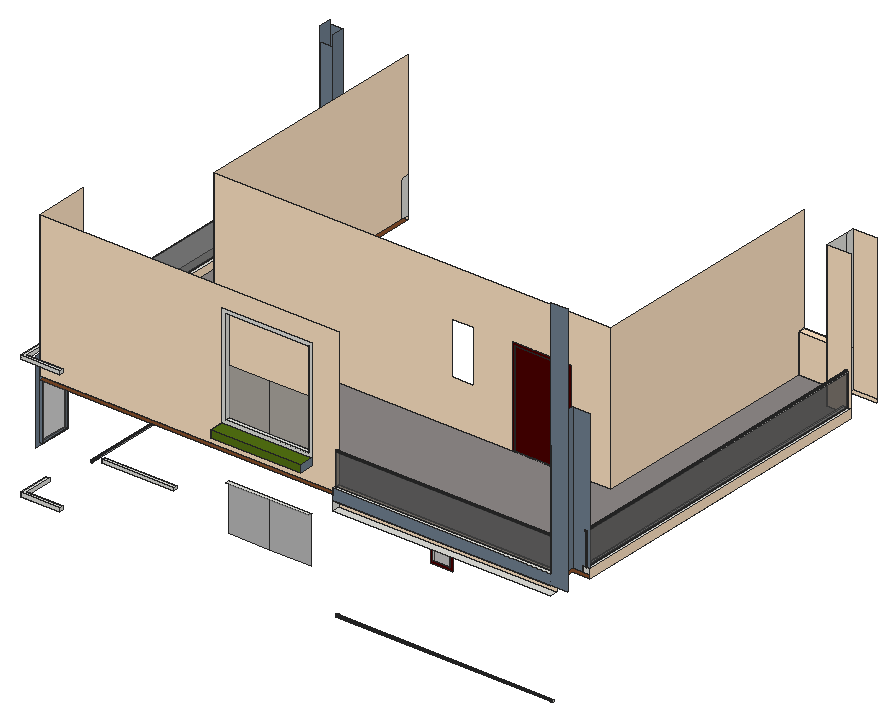
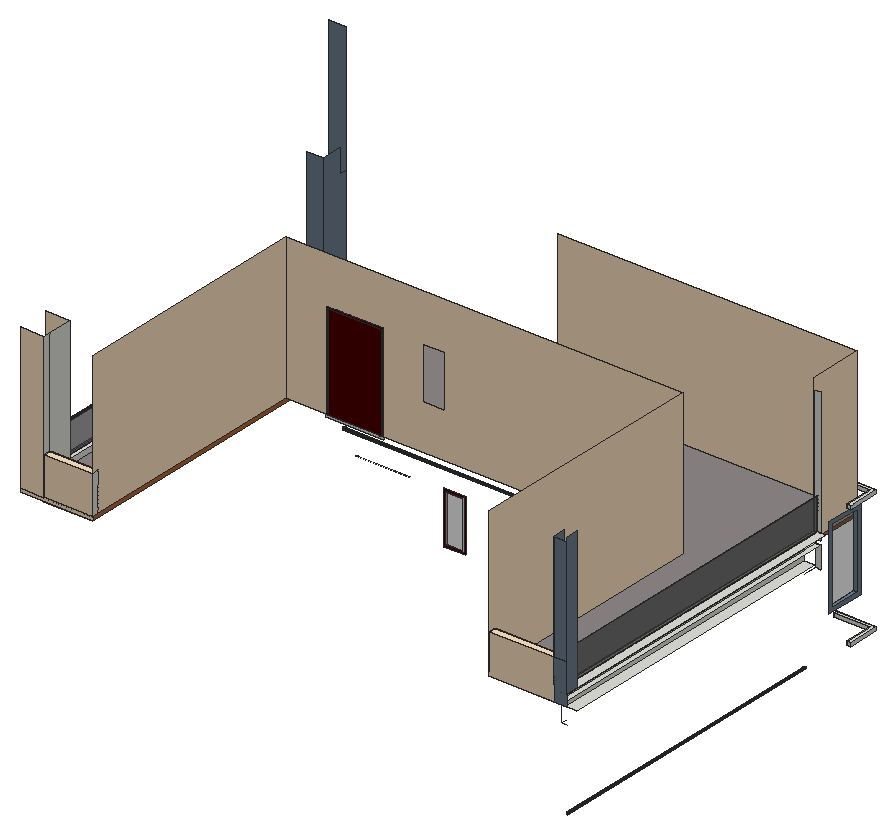
# SketchUp Ruby script. Lengths in inches.
U = 1.inch
M = Sketchup.active_model
def pt(a) = Geom::Point3d.new(a.map { |v| v * U })
def face(e, loops, mat)
  f = e.add_face(loops[0].map { |a| pt(a) })
  loops[1..].each { |l| e.add_face(l.map { |a| pt(a) }).erase! }
  f.material = f.back_material = mat if mat
  f
end
# faces: each face lists its corners as indices into pts; further lists are holes
def faces(e, pts, list, mat = nil) = list.each { |f| face(e, (f[0].is_a?(Array) ? f : [f]).map { |l| l.map { |i| pts[i] } }, mat) }
# xy, xz, yz: faces in a plane at the given z, y or x. An outline is a flat list of corners, or four numbers for a rectangle; further outlines are holes
def ring(l) = l.size == 4 ? [[l[0], l[1]], [l[2], l[1]], [l[2], l[3]], [l[0], l[3]]] : l.each_slice(2).to_a
def flat(e, list, mat, &to3) = list.each { |f| face(e, (f[0].is_a?(Array) ? f : [f]).map { |l| ring(l).map { |u, v| to3.(u, v) } }, mat) }
def xy(e, z, list, mat = nil) = flat(e, list, mat) { |x, y| [x, y, z] }
def xz(e, y, list, mat = nil) = flat(e, list, mat) { |x, z| [x, y, z] }
def yz(e, x, list, mat = nil) = flat(e, list, mat) { |y, z| [x, y, z] }
def lines(e, pts, list) = list.each { |a, b| e.add_line(pt(pts[a]), pt(pts[b])) }
# prism: a flat outline (further loops are holes) pulled along v
def prism(e, loops, v, mat = nil)
  f = face(e, loops, mat); d = Geom::Vector3d.new(v.map { |x| x * U })
  f.pushpull(f.normal.samedirection?(d) ? d.length : -d.length)
end
def box(e, o, s, mat = nil) = prism(e, [[o, [o[0] + s[0], o[1], o[2]], [o[0] + s[0], o[1] + s[1], o[2]], [o[0], o[1] + s[1], o[2]]]], [0, 0, s[2]], mat)
def at(x, y, z, deg = 0) = Geom::Transformation.translation(pt([x, y, z])) * Geom::Transformation.rotation(ORIGIN, Z_AXIS, deg.degrees)
def axes(o, x, y, z) = Geom::Transformation.new([*x, 0, *y, 0, *z, 0, *pt(o).to_a, 1])
def part(name) = M.definitions.add(name)
# library, detail: a bought-in or finely detailed component or shape, given as its bounding box
def library(name, o, s) = part(name).tap { |d| box(d.entities, o, s) }
def detail(e, o, s) = box(e.add_group.entities, o, s)
def put(e, d, t, mat = nil) = e.add_instance(d, t).tap { |i| i.material = mat if mat }
def group(e, t, mat = nil) = e.add_group.tap { |g| g.transformation = t; g.material = mat if mat }.entities
root = M.entities
M.materials.add("[0008_LavenderBlush]").color = [255, 240, 245]
M.materials.add("[0012_Bisque]").color = [255, 228, 196]
M.materials.add("[0021_DarkRed]").color = [76, 0, 0]
M.materials.add("[0111_SlateGray]").color = [112, 128, 144]
M.materials.add("[Stone Marble]").color = [143, 138, 136]
M.materials.add("[Translucent Glass Gray]").color = [84, 84, 84]
M.materials["[Translucent Glass Gray]"].alpha = 0.5
M.materials.add("[Translucent Resin Crush Gray]").color = [153, 153, 153]
M.materials["[Translucent Resin Crush Gray]"].alpha = 0.8
M.materials.add("[Vegetation Blur 03]").color = [83, 114, 18]
M.materials.add("[Wood Veneer 01]").color = [120, 70, 37]
prism(root,[[[24,204,1130.7],[24,108,1130.7],[144,108,1130.7],[144,96,1130.7],[12,96,1130.7],[12,204,1130.7]]],[0,0,12])
box(root,[282.03,96,1326.13],[240.38,12,10.37])
prism(root,[[[24,204,1539.33],[24,108,1539.33],[144,108,1539.33],[144,96,1539.33],[12,96,1539.33],[12,204,1539.33]]],[0,0,12])
xy(root,1125.03,[[35.49,360,37.49,1350]])
xy(root,1128,[[1044,118.5,1767.4375,120]])
xy(root,1152.0625,[[1088.18,468,1145.12,469.5]])
xy(root,1268.625,[[24,158.55,36,264.68]],"[0111_SlateGray]")
xy(root,1281.1,[[264,587.92,266,733.46],[264,896.41,266,1029.1875]])
xy(root,1311.1875,[[1088.18,468,1145.12,469.5]])
xy(root,1311.1875,[[1268.41,468,1446.53,469.5]],"[0021_DarkRed]")
xy(root,1411.55,[[695.08,96,971.45,108]])
xy(root,1445.3125,[[6,360,42,1350]])
xy(root,1446,[[1044,108,1767.4375,132]])
xy(root,1476,[[1044,108,1767.4375,132],[24,312,42,1368],[42,312,48,360],[147.16,473.03,144.125,473.82,141.4,475.37,139.17,477.57,137.58,480.27,136.75,483.29,136.73,486.42,137.51,489.45,139.06,492.18,141.26,494.41,143.96,495.99,146.98,496.83,150.11,496.85,153.14,496.0625,155.87,494.52,158.1,492.32,159.6875,489.62,160.52,486.6,160.54,483.47,159.76,480.4375,158.21,477.71,156.01,475.48,153.3125,473.89,150.29,473.06],[147.16,617.03,144.125,617.82,141.4,619.37,139.17,621.57,137.58,624.27,136.75,627.29,136.73,630.42,137.51,633.45,139.06,636.18,141.26,638.41,143.96,639.99,146.98,640.83,150.11,640.85,153.14,640.0625,155.87,638.52,158.1,636.32,159.6875,633.62,160.52,630.6,160.54,627.47,159.76,624.4375,158.21,621.71,156.01,619.48,153.3125,617.89,150.29,617.06],
  [147.16,761.03,144.125,761.82,141.4,763.37,139.17,765.57,137.58,768.27,136.75,771.29,136.73,774.42,137.51,777.45,139.06,780.18,141.26,782.41,143.96,783.99,146.98,784.83,150.11,784.85,153.14,784.0625,155.87,782.52,158.1,780.32,159.6875,777.62,160.52,774.6,160.54,771.47,159.76,768.4375,158.21,765.71,156.01,763.48,153.3125,761.89,150.29,761.06],[147.16,905.03,144.125,905.82,141.4,907.37,139.17,909.57,137.58,912.27,136.75,915.29,136.73,918.42,137.51,921.45,139.06,924.18,141.26,926.41,143.96,927.99,146.98,928.83,150.11,928.85,153.14,928.0625,155.87,926.52,158.1,924.32,159.6875,921.62,160.52,918.6,160.54,915.47,159.76,912.4375,158.21,909.71,156.01,907.48,153.3125,905.89,150.29,905.06],[147.16,1049.03,144.125,1049.82,141.4,1051.37,139.17,1053.57,137.58,1056.27,136.75,1059.29,136.73,1062.42,137.51,1065.45,139.06,1068.18,141.26,1070.41,143.96,1071.99,146.98,1072.83,150.11,1072.85,153.14,1072.0625,155.87,1070.52,158.1,1068.32,159.6875,1065.62,160.52,1062.6,160.54,1059.47,159.76,1056.4375,158.21,1053.71,156.01,1051.48,153.3125,1049.89,150.29,1049.06],[147.16,1193.03,144.125,1193.82,141.4,1195.37,139.17,1197.57,137.58,1200.27,136.75,1203.29,136.73,1206.42,137.51,1209.45,139.06,1212.18,141.26,1214.41,143.96,1215.99,146.98,1216.83,150.11,1216.85,153.14,1216.0625,155.87,1214.52,158.1,1212.32,159.6875,1209.62,160.52,1206.6,160.54,1203.47,159.76,1200.4375,158.21,1197.71,156.01,1195.48,153.3125,1193.89,150.29,1193.06],[42,1350,42,1368,24,1368,24,1392,48,1392,48,1350]])
xy(root,1476,[[1083.25,290.24,1077.02,290.86,1071.16,293.07,1066.07,296.73,1062.1,301.58,1059.52,307.29,1058.51,313.47,1059.13,319.7,1061.34,325.5625,1065,330.65,1069.85,334.62,1075.55,337.2,1081.74,338.21,1087.97,337.59,1093.83,335.38,1098.92,331.72,1102.89,326.875,1105.47,321.17,1106.48,314.98,1105.86,308.75,1103.65,302.89,1099.99,297.8,1095.15,293.83,1089.4375,291.25],[1359.25,290.24,1353.02,290.86,1347.16,293.07,1342.07,296.73,1338.1,301.58,1335.52,307.29,1334.51,313.47,1335.13,319.7,1337.34,325.5625,1341,330.65,1345.85,334.62,1351.55,337.2,1357.74,338.21,1363.97,337.59,1369.83,335.38,1374.92,331.72,1378.89,326.875,1381.47,321.17,1382.48,314.98,1381.86,308.75,1379.65,302.89,1375.99,297.8,1371.15,293.83,1365.4375,291.25],[1635.25,290.24,1629.02,290.86,1623.16,293.07,1618.07,296.73,1614.1,301.58,1611.52,307.29,1610.51,313.47,1611.13,319.7,1613.34,325.5625,1617,330.65,1621.85,334.62,1627.55,337.2,1633.74,338.21,1639.97,337.59,1645.83,335.38,1650.92,331.72,1654.89,326.875,1657.47,321.17,1658.48,314.98,1657.86,308.75,1655.65,302.89,1651.99,297.8,1647.15,293.83,1641.4375,291.25],[1710.75,641.49,1704.54,642.31,1698.75,644.71,1693.78,648.52,1689.97,653.49,1687.57,659.28,1686.75,665.49,1687.57,671.7,1689.97,677.49,1693.78,682.46,1698.75,686.27,1704.54,688.67,1710.75,689.49,1716.96,688.67,1722.75,686.27,1727.72,682.46,1731.54,677.49,1733.93,671.7,1734.75,665.49,1733.93,659.28,1731.54,653.49,1727.72,648.52,1722.75,644.71,1716.96,642.31],[1710.75,1078.8,1704.54,1079.62,1698.75,1082.02,1693.78,1085.83,1689.97,1090.8,1687.57,1096.59,1686.75,1102.8,1687.57,1109.01,1689.97,1114.8,1693.78,1119.77,1698.75,1123.59,1704.54,1125.99,1710.75,1126.8,1716.96,1125.99,1722.75,1123.59,1727.72,1119.77,1731.54,1114.8,1733.93,1109.01,1734.75,1102.8,1733.93,1096.59,1731.54,1090.8,1727.72,1085.83,1722.75,1082.02,1716.96,1079.62]],"[0008_LavenderBlush]")
xy(root,1476,[[[48,132,48,360,42,360,42,1350,48,1350,48,1392,264,1392,264,468,1584,468,1584,1392,1745,1392,1745,1284,1824,1284,1824,906,1745,906,1745,798,1824,798,1824,199.52,1767.4375,199.52,1767.4375,132],[1083.25,290.24,1089.4375,291.25,1095.15,293.83,1099.99,297.8,1103.65,302.89,1105.86,308.75,1106.48,314.98,1105.47,321.17,1102.89,326.875,1098.92,331.72,1093.83,335.38,1087.97,337.59,1081.74,338.21,1075.55,337.2,1069.85,334.62,1065,330.65,1061.34,325.5625,1059.13,319.7,1058.51,313.47,1059.52,307.29,1062.1,301.58,1066.07,296.73,1071.16,293.07,1077.02,290.86],[1359.25,290.24,1365.4375,291.25,1371.15,293.83,1375.99,297.8,1379.65,302.89,1381.86,308.75,1382.48,314.98,1381.47,321.17,1378.89,326.875,1374.92,331.72,1369.83,335.38,1363.97,337.59,1357.74,338.21,1351.55,337.2,1345.85,334.62,1341,330.65,1337.34,325.5625,1335.13,319.7,1334.51,313.47,1335.52,307.29,1338.1,301.58,1342.07,296.73,1347.16,293.07,1353.02,290.86],[1710.75,641.49,1716.96,642.31,1722.75,644.71,1727.72,648.52,1731.54,653.49,1733.93,659.28,1734.75,665.49,1733.93,671.7,1731.54,677.49,1727.72,682.46,1722.75,686.27,1716.96,688.67,1710.75,689.49,1704.54,688.67,1698.75,686.27,1693.78,682.46,1689.97,677.49,1687.57,671.7,1686.75,665.49,1687.57,659.28,1689.97,653.49,1693.78,648.52,1698.75,644.71,1704.54,642.31],[1710.75,1078.8,1716.96,1079.62,1722.75,1082.02,1727.72,1085.83,1731.54,1090.8,1733.93,1096.59,1734.75,1102.8,1733.93,1109.01,1731.54,1114.8,1727.72,1119.77,1722.75,1123.59,1716.96,1125.99,1710.75,1126.8,1704.54,1125.99,1698.75,1123.59,1693.78,1119.77,1689.97,1114.8,1687.57,1109.01,1686.75,1102.8,1687.57,1096.59,1689.97,1090.8,1693.78,1085.83,1698.75,1082.02,1704.54,1079.62],[1635.25,290.24,1641.4375,291.25,1647.15,293.83,1651.99,297.8,1655.65,302.89,1657.86,308.75,1658.48,314.98,1657.47,321.17,1654.89,326.875,1650.92,331.72,1645.83,335.38,1639.97,337.59,1633.74,338.21,1627.55,337.2,1621.85,334.62,1617,330.65,1613.34,325.5625,1611.13,319.7,1610.51,313.47,1611.52,307.29,1614.1,301.58,1618.07,296.73,1623.16,293.07,1629.02,290.86],[147.16,1049.03,150.29,1049.06,153.3125,1049.89,156.01,1051.48,158.21,1053.71,159.76,1056.4375,160.54,1059.47,160.52,1062.6,159.6875,1065.62,158.1,1068.32,155.87,1070.52,153.14,1072.0625,150.11,1072.85,146.98,1072.83,143.96,1071.99,141.26,1070.41,139.06,1068.18,137.51,1065.45,136.73,1062.42,136.75,1059.29,137.58,1056.27,139.17,1053.57,141.4,1051.37,144.125,1049.82],[147.16,905.03,150.29,905.06,153.3125,905.89,156.01,907.48,158.21,909.71,159.76,912.4375,160.54,915.47,160.52,918.6,159.6875,921.62,158.1,924.32,155.87,926.52,153.14,928.0625,150.11,928.85,146.98,928.83,143.96,927.99,141.26,926.41,139.06,924.18,137.51,921.45,136.73,918.42,136.75,915.29,137.58,912.27,139.17,909.57,141.4,907.37,144.125,905.82],[147.16,761.03,150.29,761.06,153.3125,761.89,156.01,763.48,158.21,765.71,159.76,768.4375,160.54,771.47,160.52,774.6,159.6875,777.62,158.1,780.32,155.87,782.52,153.14,784.0625,150.11,784.85,146.98,784.83,143.96,783.99,141.26,782.41,139.06,780.18,137.51,777.45,136.73,774.42,136.75,771.29,137.58,768.27,139.17,765.57,141.4,763.37,144.125,761.82],[147.16,617.03,150.29,617.06,153.3125,617.89,156.01,619.48,158.21,621.71,159.76,624.4375,160.54,627.47,160.52,630.6,159.6875,633.62,158.1,636.32,155.87,638.52,153.14,640.0625,150.11,640.85,146.98,640.83,143.96,639.99,141.26,638.41,139.06,636.18,137.51,633.45,136.73,630.42,136.75,627.29,137.58,624.27,139.17,621.57,141.4,619.37,144.125,617.82],[147.16,473.03,150.29,473.06,153.3125,473.89,156.01,475.48,158.21,477.71,159.76,480.4375,160.54,483.47,160.52,486.6,159.6875,489.62,158.1,492.32,155.87,494.52,153.14,496.0625,150.11,496.85,146.98,496.83,143.96,495.99,141.26,494.41,139.06,492.18,137.51,489.45,136.73,486.42,136.75,483.29,137.58,480.27,139.17,477.57,141.4,475.37,144.125,473.82],[147.16,1193.03,150.29,1193.06,153.3125,1193.89,156.01,1195.48,158.21,1197.71,159.76,1200.4375,160.54,1203.47,160.52,1206.6,159.6875,1209.62,158.1,1212.32,155.87,1214.52,153.14,1216.0625,150.11,1216.85,146.98,1216.83,143.96,1215.99,141.26,1214.41,139.06,1212.18,137.51,1209.45,136.73,1206.42,136.75,1203.29,137.58,1200.27,139.17,1197.57,141.4,1195.37,144.125,1193.82]]],"[Wood Veneer 01]")
xy(root,1488,[[1263.97,588,1442.1,589.5],[1584,1368,1745,1392]])
xy(root,1488,[[48,132,1767.4375,132,1767.4375,199.52,1800,199.52,1800,1284,1745,1284,1745,1368,1584,1368,1584,588,264,588,264,1368,48,1368]],"[Stone Marble]")
xy(root,1506,[[1800,199.52,1812,1284],[1812,199.52,1814,1284],[1814,199.52,1824,1284]])
xy(root,1512,[[1044,108,1767.4375,118.5],[1044,118.5,1767.4375,120],[6,312,34,1350],[34,312,36,1350],[36,312,48,1350]])
xy(root,1512,[[1044,120,1767.4375,132]],"[0012_Bisque]")
xy(root,1518.625,[[24,158.55,36,264.68]],"[0111_SlateGray]")
xy(root,1562.74,[[683.08,48,983.45,96]],"[0111_SlateGray]")
xy(root,1586.74,[[683.08,48,983.45,96]],"[Vegetation Blur 03]")
xy(root,1598.74,[[695.08,96,971.45,108]])
xy(root,1608,[[48,1368,264,1392]],"[0012_Bisque]")
xy(root,1611,[[1812,199.52,1814,1284]])
xy(root,1615.5,[[1584,1368,1745,1392]],"[0012_Bisque]")
xy(root,1617,[[1044,118.5,1767.4375,120]])
xy(root,1620,[[34,312,36,1350]])
xz(root,48,[[683.08,1562.74,983.45,1586.74]],"[Vegetation Blur 03]")
xz(root,96,[[[683.08,1586.74,983.45,1928.49],[695.08,1598.74,971.45,1916.49]]])
xz(root,108,[[1044,1476,1824,1476,1824,2319.6,1767.4375,2319.6,1767.4375,1512,1044,1512]],"[0111_SlateGray]")
xz(root,108,[[695.08,1252.68,833.27,1411.55],[833.27,1252.68,971.45,1411.55],[695.08,1598.74,833.27,1757.62],[833.27,1598.74,971.45,1757.62]],"[Translucent Resin Crush Gray]")
xz(root,118.5,[[1044,1512,1767.4375,1617]],"[Translucent Glass Gray]")
xz(root,120,[[1044,1617,1767.4375,1620]])
xz(root,120,[[1044,1512,1767.4375,1617]],"[Translucent Glass Gray]")
xz(root,132,[[1044,1446,1767.4375,1476],[48,1488,1044,1968],[1044,1488,1767.4375,1512]],"[0012_Bisque]")
xz(root,158.55,[[24,1268.625,36,1518.625]],"[0111_SlateGray]")
xz(root,199.52,[[1800,1488,1824,1506],[1812,1506,1814,1611]])
xz(root,199.52,[[[1767.4375,1488,1767.4375,1968,1824,1968,1824,1506,1800,1506,1800,1488],[1812,1611,1812.3125,1611.02,1812.625,1611.07,1812.93,1611.15,1813.22,1611.26,1813.5,1611.4,1813.76,1611.57,1814.01,1611.77,1814.23,1611.99,1814.43,1612.24,1814.6,1612.5,1814.74,1612.78,1814.85,1613.07,1814.93,1613.375,1814.98,1613.6875,1815,1614,1814.98,1614.3125,1814.93,1614.625,1814.85,1614.93,1814.74,1615.22,1814.6,1615.5,1814.43,1615.76,1814.23,1616.01,1814.01,1616.23,1813.76,1616.43,1813.5,1616.6,1813.22,1616.74,1812.93,1616.85,1812.625,1616.93,1812.3125,1616.98,1812,1617,1811.6875,1616.98,1811.375,1616.93,1811.07,1616.85,1810.78,1616.74,1810.5,1616.6,1810.24,1616.43,1809.99,1616.23,1809.77,1616.01,1809.57,1615.76,1809.4,1615.5,1809.26,1615.22,1809.15,1614.93,1809.07,1614.625,1809.02,1614.3125,1809,1614,1809.02,1613.6875,1809.07,1613.375,1809.15,1613.07,1809.26,1612.78,1809.4,1612.5,1809.57,1612.24,1809.77,1611.99,1809.99,1611.77,1810.24,1611.57,1810.5,1611.4,1810.78,1611.26,1811.07,1611.15,1811.375,1611.07,1811.6875,1611.02]]],"[0111_SlateGray]")
xz(root,264.68,[[24,1268.625,36,1518.625]],"[0111_SlateGray]")
xz(root,312,[[24,1404,42,1476],[24,1488,48,1512],[24,1512,24,1932,48,1932,48,1512,36,1512,36,1620,34,1620,34,1512],[34,1512,36,1572],[34,1572,36,1620]])
xz(root,360,[[37.18,1125.02,37.49,1125.03,37.125,1125.03]])
xz(root,468,[[[1080.18,1144.0625,1153.12,1319.1875],[1088.18,1152.0625,1145.12,1311.1875]]],"[0021_DarkRed]")
xz(root,469.5,[[1088.18,1152.0625,1145.12,1311.1875]],"[Translucent Glass Gray]")
xz(root,588,[[1255.97,1480,1450.1,1488]])
xz(root,588,[[[264,1488,1255.97,1488,1255.97,1811.1875,1450.1,1811.1875,1450.1,1488,1584,1488,1584,1968,264,1968],[1053.52,1636.0625,1126.46,1811.1875]]],"[0012_Bisque]")
xz(root,588,[[1255.97,1488,1263.97,1488,1263.97,1803.1875,1442.1,1803.1875,1442.1,1488,1450.1,1488,1450.1,1811.1875,1255.97,1811.1875]],"[0021_DarkRed]")
xz(root,589.5,[[1263.97,1488,1442.1,1803.1875]],"[0021_DarkRed]")
xz(root,1284,[[1800,1488,1824,1506],[1812,1506,1814,1611],[1812,1611,1811.6875,1611.02,1811.375,1611.07,1811.07,1611.15,1810.78,1611.26,1810.5,1611.4,1810.24,1611.57,1809.99,1611.77,1809.77,1611.99,1809.57,1612.24,1809.4,1612.5,1809.26,1612.78,1809.15,1613.07,1809.07,1613.375,1809.02,1613.6875,1809,1614,1809.02,1614.3125,1809.07,1614.625,1809.15,1614.93,1809.26,1615.22,1809.4,1615.5,1809.57,1615.76,1809.77,1616.01,1809.99,1616.23,1810.24,1616.43,1810.5,1616.6,1810.78,1616.74,1811.07,1616.85,1811.375,1616.93,1811.6875,1616.98,1812,1617,1812.3125,1616.98,1812.625,1616.93,1812.93,1616.85,1813.22,1616.74,1813.5,1616.6,1813.76,1616.43,1814.01,1616.23,1814.23,1616.01,1814.43,1615.76,1814.6,1615.5,1814.74,1615.22,1814.85,1614.93,1814.93,1614.625,1814.98,1614.3125,1815,1614,1814.98,1613.6875,1814.93,1613.375,1814.85,1613.07,1814.74,1612.78,1814.6,1612.5,1814.43,1612.24,1814.23,1611.99,1814.01,1611.77,1813.76,1611.57,1813.5,1611.4,1813.22,1611.26,1812.93,1611.15,1812.625,1611.07,1812.3125,1611.02]])
xz(root,1284,[[[1745,1488,1800,1488,1800,1506,1824,1506,1824,1968,1745,1968],[1812,1611,1811.6875,1611.02,1811.375,1611.07,1811.07,1611.15,1810.78,1611.26,1810.5,1611.4,1810.24,1611.57,1809.99,1611.77,1809.77,1611.99,1809.57,1612.24,1809.4,1612.5,1809.26,1612.78,1809.15,1613.07,1809.07,1613.375,1809.02,1613.6875,1809,1614,1809.02,1614.3125,1809.07,1614.625,1809.15,1614.93,1809.26,1615.22,1809.4,1615.5,1809.57,1615.76,1809.77,1616.01,1809.99,1616.23,1810.24,1616.43,1810.5,1616.6,1810.78,1616.74,1811.07,1616.85,1811.375,1616.93,1811.6875,1616.98,1812,1617,1812.3125,1616.98,1812.625,1616.93,1812.93,1616.85,1813.22,1616.74,1813.5,1616.6,1813.76,1616.43,1814.01,1616.23,1814.23,1616.01,1814.43,1615.76,1814.6,1615.5,1814.74,1615.22,1814.85,1614.93,1814.93,1614.625,1814.98,1614.3125,1815,1614,1814.98,1613.6875,1814.93,1613.375,1814.85,1613.07,1814.74,1612.78,1814.6,1612.5,1814.43,1612.24,1814.23,1611.99,1814.01,1611.77,1813.76,1611.57,1813.5,1611.4,1813.22,1611.26,1812.93,1611.15,1812.625,1611.07,1812.3125,1611.02]]],"[0012_Bisque]")
xz(root,1350,[[37.81,1125.02,37.49,1125.03,37.125,1125.03,36.87,1125.07,36.57,1125.15,36.27,1125.26,35.99,1125.4,35.73,1125.57,35.49,1125.77,35.26,1125.99,35.07,1126.24,34.9,1126.5,34.75,1126.78,34.64,1127.07,34.56,1127.375,34.51,1127.6875,34.49,1128,34.51,1128.3125,34.56,1128.625,34.64,1128.93,34.75,1129.22,34.9,1129.5,35.07,1129.76,35.26,1130.01,35.49,1130.23,35.73,1130.43,35.99,1130.6,36.27,1130.74,36.57,1130.85,36.87,1130.93,37.18,1130.98,37.49,1131,37.81,1130.98,38.12,1130.93,38.42,1130.85,38.71,1130.74,38.99,1130.6,39.26,1130.43,39.5,1130.23,39.72,1130.01,39.92,1129.76,40.09,1129.5,40.24,1129.22,40.35,1128.93,40.43,1128.625,40.48,1128.3125,40.49,1128,40.48,1127.6875,40.43,1127.375,40.35,1127.07,40.24,1126.78,40.09,1126.5,39.92,1126.24,39.72,1125.99,39.5,1125.77,39.26,1125.57,38.99,1125.4,38.71,1125.26,38.42,1125.15,38.12,1125.07],[37.18,1125.02,37.125,1125.03,37.49,1125.03],[34,1512,36,1620]])
xz(root,1350,[[6,1512,34,1512,34,1620,36,1620,36,1512,48,1512,48,1932,6,1932]],"[0111_SlateGray]")
xz(root,1368,[[48,1488,264,1608],[1584,1488,1745,1615.5]],"[0012_Bisque]")
xz(root,1392,[[48,1476,264,1608],[1584,1476,1824,1488],[1584,1488,1745,1615.5],[1745,1488,1824,1968]],"[0012_Bisque]")
xz(root,1392,[[6,1476,48,1608],[6,1608,48,1968]],"[0111_SlateGray]")
yz(root,6,[[1350,1512,1392,1980]],"[0111_SlateGray]")
yz(root,24,[[[146.55,1256.625,276.68,1530.625],[158.55,1268.625,264.68,1518.625]]],"[0111_SlateGray]")
yz(root,34,[[312,1512,1350,1620]],"[Translucent Glass Gray]")
yz(root,36,[[158.55,1268.625,264.68,1518.625],[312,1512,1350,1620]],"[Translucent Glass Gray]")
yz(root,37.49,[[360,1125.03,1350,1128]])
yz(root,42,[[360,1445.3125,1350,1476]])
yz(root,48,[[1350,1512,1368,1608]])
yz(root,48,[[132,1488,312,1968],[312,1488,1368,1512]],"[0012_Bisque]")
yz(root,48,[[1350,1608,1392,1968]],"[0111_SlateGray]")
yz(root,264,[[1368,1488,1392,1608]])
yz(root,264,[[588,1488,588,1968,1392,1968,1392,1608,1368,1608,1368,1488]],"[0012_Bisque]")
yz(root,683.08,[[48,1562.74,96,1586.74]],"[0111_SlateGray]")
yz(root,695.08,[[96,1598.74,108,1916.49]])
yz(root,971.45,[[96,1598.74,108,1916.49]])
yz(root,983.45,[[48,1562.74,96,1586.74]],"[0111_SlateGray]")
yz(root,1044,[[118.5,1125.02,118.5,1125.43,118.78,1125.26,119.53,1125.04,120,1125.02],[120,1125.02,119.53,1125.04,118.78,1125.26,118.5,1125.43,118.5,1128,120,1128],[108,1446,132,1476],[108,1488,132,1512],[118.5,1512,120,1617]])
yz(root,1088.18,[[468,1152.0625,469.5,1311.1875]])
yz(root,1145.12,[[468,1152.0625,469.5,1311.1875]])
yz(root,1263.97,[[588,1488,589.5,1803.1875]],"[0021_DarkRed]")
yz(root,1442.1,[[588,1488,589.5,1803.1875]],"[0021_DarkRed]")
yz(root,1584,[[1368,1488,1392,1615.5]])
yz(root,1584,[[588,1488,1368,1488,1368,1615.5,1392,1615.5,1392,1968,588,1968]],"[0012_Bisque]")
yz(root,1745,[[1284,1488,1368,1968],[1368,1488,1392,1615.5],[1368,1615.5,1392,1968]])
yz(root,1767.4375,[[120,1125.02,120.3125,1125.02,121.08,1125.2,121.76,1125.57,122.33,1126.11,122.74,1126.78,122.96,1127.53,122.98,1128.3125,122.8,1129.08,122.43,1129.76,121.89,1130.33,121.22,1130.74,120.47,1130.96,119.6875,1130.98,118.92,1130.8,118.24,1130.43,117.67,1129.89,117.26,1129.22,117.04,1128.47,117.02,1127.6875,117.2,1126.92,117.57,1126.24,118.11,1125.67,118.5,1125.43,118.5,1128,120,1128],[118.5,1125.02,120,1125.02,119.53,1125.04,118.78,1125.26,118.5,1125.43],[120,1125.02,120,1128,118.5,1128,118.5,1125.43,118.78,1125.26,119.53,1125.04],[118.5,1512,120,1617],[120,1617,120.78,1617.1,121.5,1617.4,122.12,1617.88,122.6,1618.5,122.9,1619.22,123,1620,122.9,1620.78,122.6,1621.5,122.12,1622.12,121.5,1622.6,120.78,1622.9,120,1623,119.22,1622.9,118.5,1622.6,117.88,1622.12,117.4,1621.5,117.1,1620.78,117,1620,117.1,1619.22,117.4,1618.5,117.88,1617.88,118.5,1617.4,119.22,1617.1]])
yz(root,1767.4375,[[[132,1488,132,1512,108,1512,108,1891.5,132,1891.5,132,1968,199.52,1968,199.52,1488],[120,1617,120.78,1617.1,121.5,1617.4,122.12,1617.88,122.6,1618.5,122.9,1619.22,123,1620,122.9,1620.78,122.6,1621.5,122.12,1622.12,121.5,1622.6,120.78,1622.9,120,1623,119.22,1622.9,118.5,1622.6,117.88,1622.12,117.4,1621.5,117.1,1620.78,117,1620,117.1,1619.22,117.4,1618.5,117.88,1617.88,118.5,1617.4,119.22,1617.1]]],"[0111_SlateGray]")
yz(root,1800,[[199.52,1488,1284,1506]])
yz(root,1812,[[199.52,1611,1284,1614]])
yz(root,1812,[[199.52,1506,1284,1611]],"[Translucent Glass Gray]")
yz(root,1814,[[199.52,1506,1284,1611]],"[Translucent Glass Gray]")
yz(root,1824,[[199.52,1476,1284,1506]],"[0012_Bisque]")
p = [[1767.4375,119.53,1125.04],[1767.4375,118.78,1125.26],[1044,118.78,1125.26],[1044,119.53,1125.04],[1767.4375,120.3125,1125.02],[1767.4375,120,1125.02],
  [1044,120,1125.02],[1044,120.3125,1125.02],[1767.4375,121.08,1125.2],[1044,121.08,1125.2],[36.87,1350,1125.07],[37.125,1350,1125.03],
  [37.18,1350,1125.02],[37.18,360,1125.02],[37.125,360,1125.03],[36.87,360,1125.07],[37.49,1350,1125.03],[37.49,360,1125.03],
  [37.81,1350,1125.02],[37.81,360,1125.02],[38.12,1350,1125.07],[38.12,360,1125.07],[36.27,1350,1125.26],[36.57,1350,1125.15],
  [36.57,360,1125.15],[36.27,360,1125.26],[38.42,1350,1125.15],[38.42,360,1125.15],[38.71,1350,1125.26],[38.71,360,1125.26],
  [1767.4375,121.76,1125.57],[1044,121.76,1125.57],[1767.4375,118.5,1125.43],[1767.4375,118.11,1125.67],[1044,118.11,1125.67],[1044,118.5,1125.43],
  [35.99,1350,1125.4],[35.99,360,1125.4],[38.99,1350,1125.4],[38.99,360,1125.4],[35.73,1350,1125.57],[35.73,360,1125.57],
  [39.26,1350,1125.57],[39.26,360,1125.57],[1767.4375,122.33,1126.11],[1044,122.33,1126.11],[35.49,1350,1125.77],[35.49,360,1125.77],
  [39.5,1350,1125.77],[39.5,360,1125.77],[1767.4375,117.57,1126.24],[1044,117.57,1126.24],[35.26,1350,1125.99],[35.26,360,1125.99],
  [39.72,1350,1125.99],[39.72,360,1125.99],[35.07,1350,1126.24],[35.07,360,1126.24],[39.92,1350,1126.24],[39.92,360,1126.24],
  [1767.4375,122.74,1126.78],[1044,122.74,1126.78],[1767.4375,117.2,1126.92],[1044,117.2,1126.92],[34.9,1350,1126.5],[34.9,360,1126.5],
  [40.09,1350,1126.5],[40.09,360,1126.5],[34.75,1350,1126.78],[34.75,360,1126.78],[40.24,1350,1126.78],[40.24,360,1126.78],
  [1767.4375,122.96,1127.53],[1044,122.96,1127.53],[34.64,1350,1127.07],[34.64,360,1127.07],[40.35,1350,1127.07],[40.35,360,1127.07],
  [1767.4375,117.02,1127.6875],[1044,117.02,1127.6875],[34.56,1350,1127.375],[34.56,360,1127.375],[40.43,1350,1127.375],[40.43,360,1127.375],
  [34.51,1350,1127.6875],[34.51,360,1127.6875],[40.48,1350,1127.6875],[40.48,360,1127.6875],[1767.4375,122.98,1128.3125],[1044,122.98,1128.3125],
  [1767.4375,117.04,1128.47],[1044,117.04,1128.47],[34.49,1350,1128],[34.49,360,1128],[40.49,1350,1128],[40.49,360,1128],
  [34.51,1350,1128.3125],[34.51,360,1128.3125],[40.48,1350,1128.3125],[40.48,360,1128.3125],[1767.4375,122.8,1129.08],[1044,122.8,1129.08],
  [34.56,1350,1128.625],[34.56,360,1128.625],[40.43,1350,1128.625],[40.43,360,1128.625],[1767.4375,117.26,1129.22],[1044,117.26,1129.22],
  [34.64,1350,1128.93],[34.64,360,1128.93],[40.35,1350,1128.93],[40.35,360,1128.93],[34.75,1350,1129.22],[34.75,360,1129.22],
  [40.24,1350,1129.22],[40.24,360,1129.22],[1767.4375,122.43,1129.76],[1044,122.43,1129.76],[1767.4375,117.67,1129.89],[1044,117.67,1129.89],
  [34.9,1350,1129.5],[34.9,360,1129.5],[40.09,1350,1129.5],[40.09,360,1129.5],[35.07,1350,1129.76],[35.07,360,1129.76],
  [39.92,1350,1129.76],[39.92,360,1129.76],[1767.4375,121.89,1130.33],[1044,121.89,1130.33],[35.26,1350,1130.01],[35.26,360,1130.01],
  [39.72,1350,1130.01],[39.72,360,1130.01],[1767.4375,118.24,1130.43],[1044,118.24,1130.43],[35.49,1350,1130.23],[35.49,360,1130.23],
  [39.5,1350,1130.23],[39.5,360,1130.23],[35.73,1350,1130.43],[35.73,360,1130.43],[39.26,1350,1130.43],[39.26,360,1130.43],
  [1767.4375,121.22,1130.74],[1044,121.22,1130.74],[1767.4375,118.92,1130.8],[1044,118.92,1130.8],[35.99,1350,1130.6],[35.99,360,1130.6],
  [38.99,1350,1130.6],[38.99,360,1130.6],[36.27,1350,1130.74],[36.27,360,1130.74],[38.71,1350,1130.74],[38.71,360,1130.74],
  [1767.4375,120.47,1130.96],[1044,120.47,1130.96],[36.57,1350,1130.85],[36.57,360,1130.85],[38.42,1350,1130.85],[38.42,360,1130.85],
  [1767.4375,119.6875,1130.98],[1044,119.6875,1130.98],[36.87,1350,1130.93],[36.87,360,1130.93],[37.18,1350,1130.98],[37.18,360,1130.98],
  [38.12,1350,1130.93],[37.81,1350,1130.98],[37.81,360,1130.98],[38.12,360,1130.93],[37.49,1350,1131],[37.49,360,1131],
  [1811.375,1284,1611.07],[1811.6875,1284,1611.02],[1811.6875,199.52,1611.02],[1811.375,199.52,1611.07],[1812,1284,1611],[1812,199.52,1611],
  [1812.3125,1284,1611.02],[1812.3125,199.52,1611.02],[1812.625,1284,1611.07],[1812.625,199.52,1611.07],[1810.78,1284,1611.26],[1811.07,1284,1611.15],
  [1811.07,199.52,1611.15],[1810.78,199.52,1611.26],[1812.93,1284,1611.15],[1812.93,199.52,1611.15],[1813.22,1284,1611.26],[1813.22,199.52,1611.26],
  [1810.5,1284,1611.4],[1810.5,199.52,1611.4],[1813.5,1284,1611.4],[1813.5,199.52,1611.4],[1810.24,1284,1611.57],[1810.24,199.52,1611.57],
  [1813.76,1284,1611.57],[1813.76,199.52,1611.57],[1809.99,1284,1611.77],[1809.99,199.52,1611.77],[1814.01,1284,1611.77],[1814.01,199.52,1611.77],
  [1809.77,1284,1611.99],[1809.77,199.52,1611.99],[1814.23,1284,1611.99],[1814.23,199.52,1611.99],[1809.57,1284,1612.24],[1809.57,199.52,1612.24],
  [1814.43,1284,1612.24],[1814.43,199.52,1612.24],[1809.4,1284,1612.5],[1809.4,199.52,1612.5],[1814.6,1284,1612.5],[1814.6,199.52,1612.5],
  [1809.26,1284,1612.78],[1809.26,199.52,1612.78],[1814.74,1284,1612.78],[1814.74,199.52,1612.78],[1809.15,1284,1613.07],[1809.15,199.52,1613.07],
  [1814.85,1284,1613.07],[1814.85,199.52,1613.07],[1809.07,1284,1613.375],[1809.07,199.52,1613.375],[1814.93,1284,1613.375],[1814.93,199.52,1613.375],
  [1809.02,1284,1613.6875],[1809.02,199.52,1613.6875],[1814.98,1284,1613.6875],[1814.98,199.52,1613.6875],[1809,1284,1614],[1809,199.52,1614],
  [1815,1284,1614],[1815,199.52,1614],[1809.02,1284,1614.3125],[1809.02,199.52,1614.3125],[1814.98,1284,1614.3125],[1814.98,199.52,1614.3125],
  [1809.07,1284,1614.625],[1809.07,199.52,1614.625],[1814.93,1284,1614.625],[1814.93,199.52,1614.625],[1809.15,1284,1614.93],[1809.15,199.52,1614.93],
  [1814.85,1284,1614.93],[1814.85,199.52,1614.93],[1809.26,1284,1615.22],[1809.26,199.52,1615.22],[1814.74,1284,1615.22],[1814.74,199.52,1615.22],
  [1809.4,1284,1615.5],[1809.4,199.52,1615.5],[1814.6,1284,1615.5],[1814.6,199.52,1615.5],[1809.57,1284,1615.76],[1809.57,199.52,1615.76],
  [1814.43,1284,1615.76],[1814.43,199.52,1615.76],[1809.77,1284,1616.01],[1809.77,199.52,1616.01],[1814.23,1284,1616.01],[1814.23,199.52,1616.01],
  [1809.99,1284,1616.23],[1809.99,199.52,1616.23],[1814.01,1284,1616.23],[1814.01,199.52,1616.23],[1810.24,1284,1616.43],[1810.24,199.52,1616.43],
  [1813.76,1284,1616.43],[1813.76,199.52,1616.43],[1810.5,1284,1616.6],[1810.5,199.52,1616.6],[1813.5,1284,1616.6],[1813.5,199.52,1616.6],
  [1810.78,1284,1616.74],[1810.78,199.52,1616.74],[1813.22,1284,1616.74],[1813.22,199.52,1616.74],[1811.07,1284,1616.85],[1811.07,199.52,1616.85],
  [1812.93,1284,1616.85],[1812.93,199.52,1616.85],[1811.375,1284,1616.93],[1811.375,199.52,1616.93],[1811.6875,1284,1616.98],[1811.6875,199.52,1616.98],
  [1812.625,1284,1616.93],[1812.3125,1284,1616.98],[1812.3125,199.52,1616.98],[1812.625,199.52,1616.93],[1767.4375,120,1617],[1767.4375,119.22,1617.1],
  [1044,119.22,1617.1],[1044,120,1617],[1767.4375,120.78,1617.1],[1044,120.78,1617.1],[1812,1284,1617],[1812,199.52,1617],
  [1767.4375,118.5,1617.4],[1044,118.5,1617.4],[1767.4375,121.5,1617.4],[1044,121.5,1617.4],[1767.4375,117.88,1617.88],[1044,117.88,1617.88],
  [1767.4375,122.12,1617.88],[1044,122.12,1617.88],[1767.4375,117.4,1618.5],[1044,117.4,1618.5],[1767.4375,122.6,1618.5],[1044,122.6,1618.5],
  [1767.4375,117.1,1619.22],[1044,117.1,1619.22],[1767.4375,122.9,1619.22],[1044,122.9,1619.22],[1767.4375,117,1620],[1044,117,1620],
  [1767.4375,123,1620],[1044,123,1620],[1767.4375,117.1,1620.78],[1044,117.1,1620.78],[1767.4375,122.9,1620.78],[1044,122.9,1620.78],
  [1767.4375,117.4,1621.5],[1044,117.4,1621.5],[1767.4375,122.6,1621.5],[1044,122.6,1621.5],[48,1368,1488],[24,1368,1488],
  [42,1368,1404],[24,1368,1404],[42,312,1404],[42,360,1404],[42,1368,1476],[42,1350,1404],
  [24,1368,1512],[24,1392,1512],[24,1368,1476],[1767.4375,132,1488],[1767.4375,108,1488],[6,1368,1512]]
faces(root,p,[[0,1,2,3],[4,5,0,3,6,7],[8,4,7,9],[10,11,12,13,14,15],[12,16,17,13],[16,18,19,17],[18,20,21,19],[22,23,24,25],
  [23,10,15,24],[20,26,27,21],[26,28,29,27],[30,8,9,31],[1,32,33,34,35,2],[36,22,25,37],[28,38,39,29],[40,36,37,41],
  [38,42,43,39],[44,30,31,45],[46,40,41,47],[42,48,49,43],[33,50,51,34],[52,46,47,53],[48,54,55,49],[56,52,53,57],
  [54,58,59,55],[60,44,45,61],[50,62,63,51],[64,56,57,65],[58,66,67,59],[68,64,65,69],[66,70,71,67],[72,60,61,73],
  [74,68,69,75],[70,76,77,71],[62,78,79,63],[80,74,75,81],[76,82,83,77],[84,80,81,85],[82,86,87,83],[88,72,73,89],
  [78,90,91,79],[92,84,85,93],[86,94,95,87],[96,92,93,97],[94,98,99,95],[100,88,89,101],[102,96,97,103],[98,104,105,99],
  [90,106,107,91],[108,102,103,109],[104,110,111,105],[112,108,109,113],[110,114,115,111],[116,100,101,117],[106,118,119,107],[120,112,113,121],
  [114,122,123,115],[124,120,121,125],[122,126,127,123],[128,116,117,129],[130,124,125,131],[126,132,133,127],[118,134,135,119],[136,130,131,137],
  [132,138,139,133],[140,136,137,141],[138,142,143,139],[144,128,129,145],[134,146,147,135],[148,140,141,149],[142,150,151,143],[152,148,149,153],
  [150,154,155,151],[156,144,145,157],[158,152,153,159],[154,160,161,155],[146,162,163,147],[164,158,159,165],[166,164,165,167],[168,169,170,171],
  [160,168,171,161],[162,156,157,163],[172,166,167,173],[169,172,173,170],[174,175,176,177],[175,178,179,176],[178,180,181,179],[180,182,183,181],
  [184,185,186,187],[185,174,177,186],[182,188,189,183],[188,190,191,189],[192,184,187,193],[190,194,195,191],[196,192,193,197],[194,198,199,195],
  [200,196,197,201],[198,202,203,199],[204,200,201,205],[202,206,207,203],[208,204,205,209],[206,210,211,207],[212,208,209,213],[210,214,215,211],
  [216,212,213,217],[214,218,219,215],[220,216,217,221],[218,222,223,219],[224,220,221,225],[222,226,227,223],[228,224,225,229],[226,230,231,227],
  [232,228,229,233],[230,234,235,231],[236,232,233,237],[234,238,239,235],[240,236,237,241],[238,242,243,239],[244,240,241,245],[242,246,247,243],
  [248,244,245,249],[246,250,251,247],[252,248,249,253],[250,254,255,251],[256,252,253,257],[254,258,259,255],[260,256,257,261],[258,262,263,259],
  [264,260,261,265],[262,266,267,263],[268,264,265,269],[266,270,271,267],[272,268,269,273],[270,274,275,271],[276,272,273,277],[274,278,279,275],
  [280,276,277,281],[278,282,283,279],[284,280,281,285],[286,284,285,287],[288,289,290,291],[282,288,291,283],[292,293,294,295],[296,292,295,297],
  [298,286,287,299],[289,298,299,290],[293,300,301,294],[302,296,297,303],[300,304,305,301],[306,302,303,307],[304,308,309,305],[310,306,307,311],
  [308,312,313,309],[314,310,311,315],[312,316,317,313],[318,314,315,319],[316,320,321,317],[322,318,319,323],[320,324,325,321],[326,322,323,327]])
lines(root,p,[[328,329],[330,331],[332,333],[334,330],[335,330],[336,337],[338,329],[329,336],[339,340],[336,341]])
